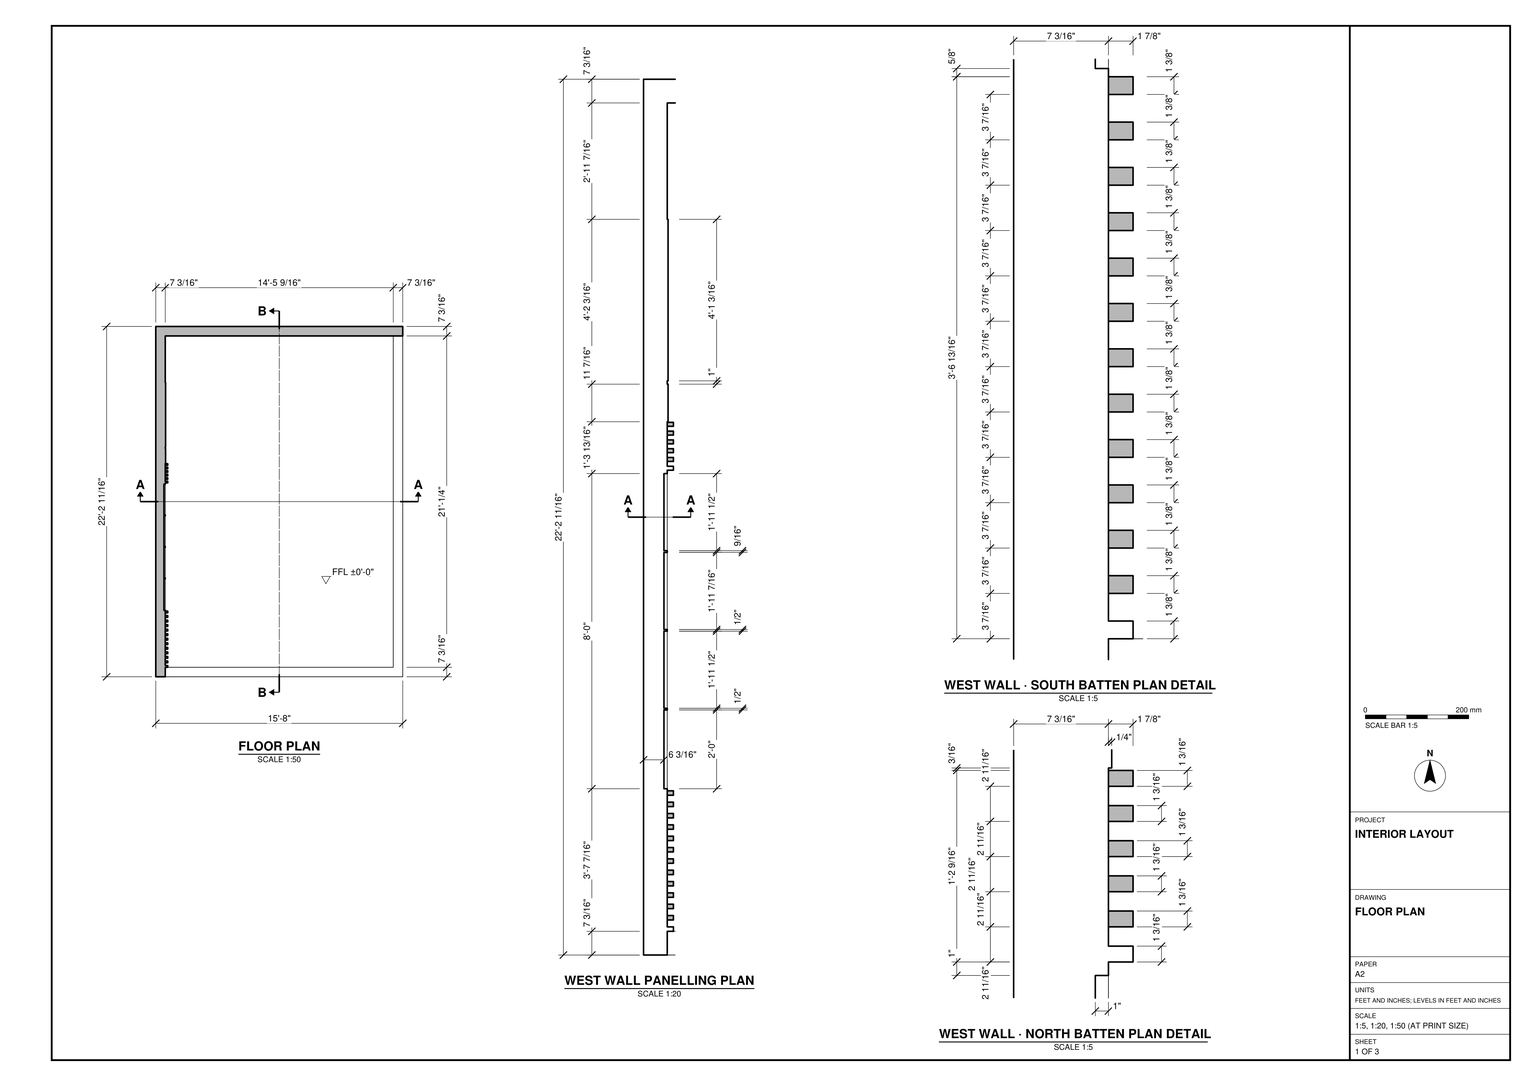
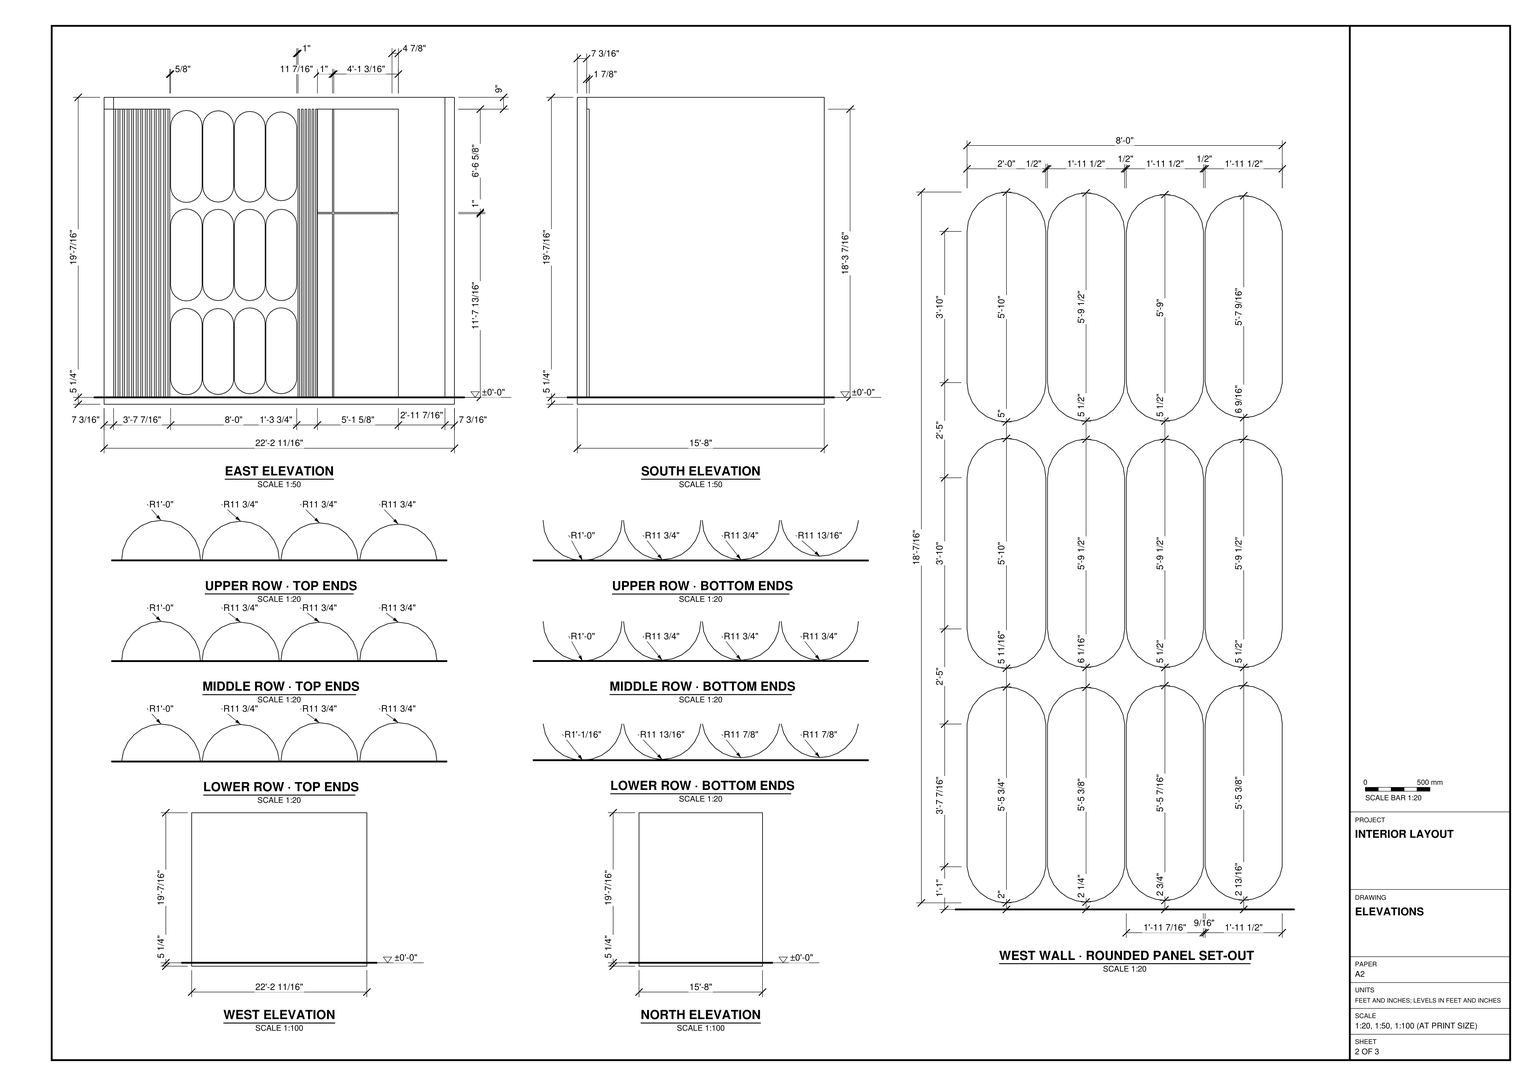
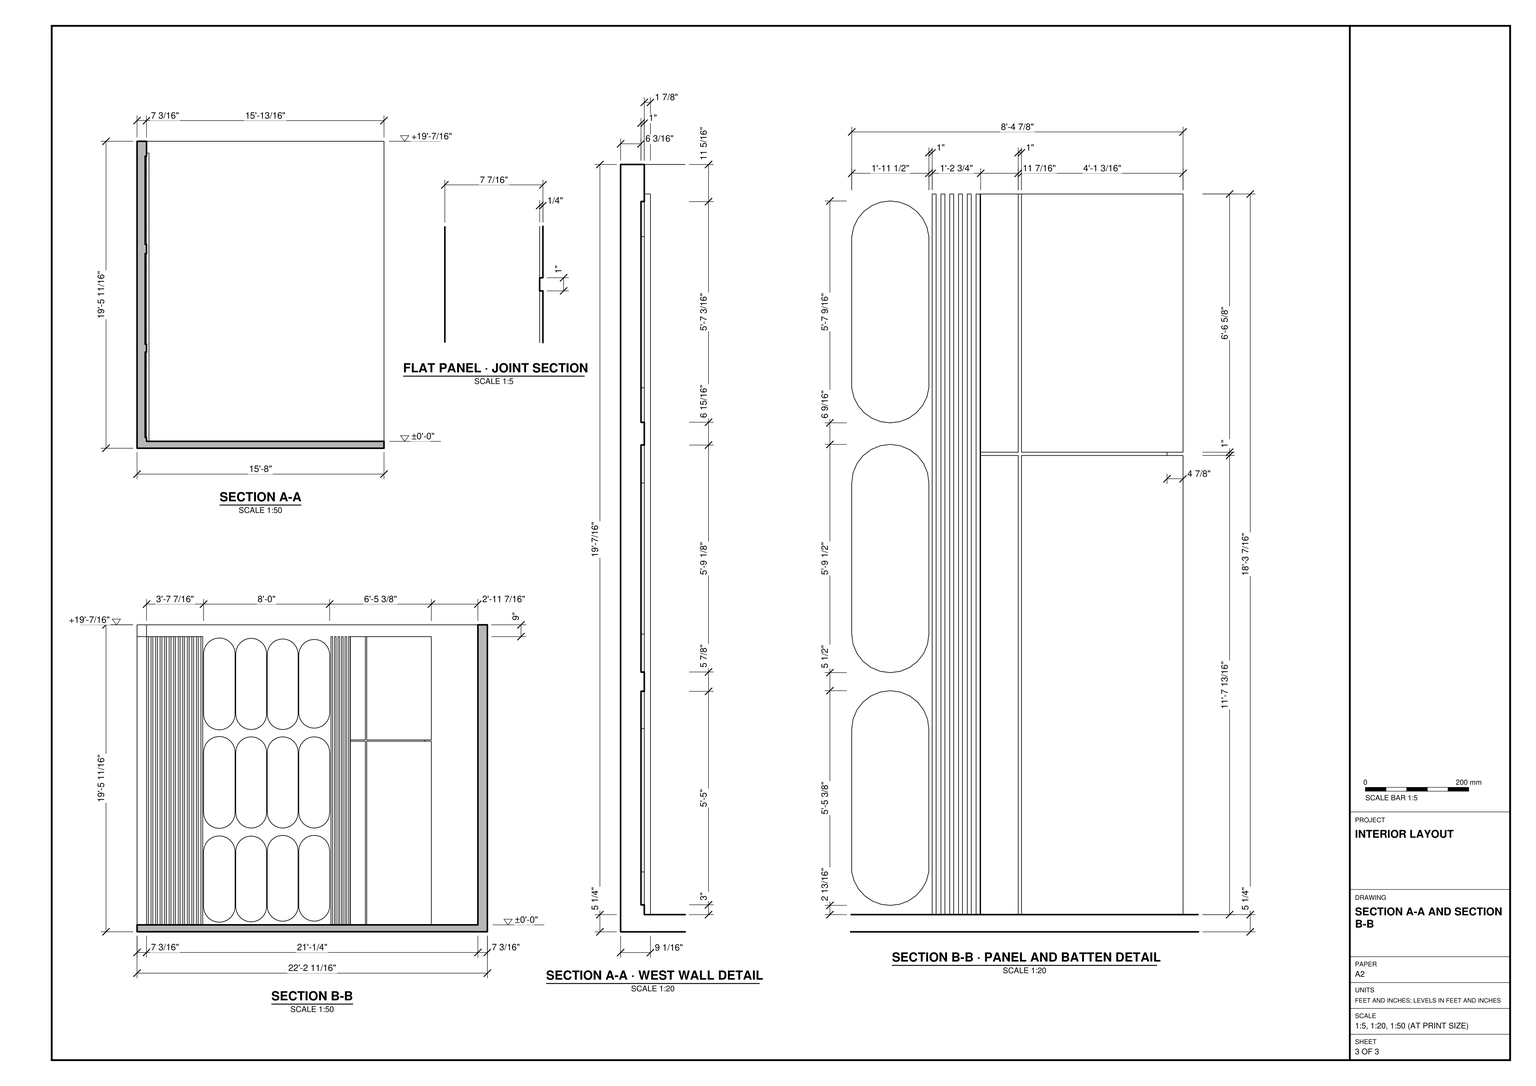
Build the interior shown in task_files/diagram_01.pdf in SketchUp. Work in feet and inches. Set the finished floor at ±0'-0" and model the rectangular slab with the west wall along its long edge and the north wall returning across its short edge. The overall dimensions are 15'-8" east to west, 22'-2 11/16" north to south and 19'-5 11/16" from the underside of the slab to the top of the walls. Make the slab 5 1/4" thick and use the 7 3/16" wall thickness shown in plan.

Set out the panelling on the room side of the west wall. Working from south to north, model the wider batten field, the rounded panels, the narrower batten field and the flat panels, leaving the plain wall face visible at the north end. Follow the separate plan details for the two batten spacings. Use the elevation to lay out the rounded ends in four columns and three rows, and use the sections to form the changes in face depth and the joints between flat panels.

Keep the slab, walls and built-in panelling in separate groups or components, and use components for repeated parts. Any decor or loose items shown may be suitable library components. Save one SketchUp model as output_files/interior_corner_with_detailed_west_wall_panelling.skp.

# SketchUp Ruby script. Lengths in inches.
U = 1.inch
M = Sketchup.active_model
def pt(a) = Geom::Point3d.new(a.map { |v| v * U })
def face(e, loops, mat)
  f = e.add_face(loops[0].map { |a| pt(a) })
  loops[1..].each { |l| e.add_face(l.map { |a| pt(a) }).erase! }
  f.material = f.back_material = mat if mat
  f
end
# faces: each face lists its corners as indices into pts; further lists are holes
def faces(e, pts, list, mat = nil) = list.each { |f| face(e, (f[0].is_a?(Array) ? f : [f]).map { |l| l.map { |i| pts[i] } }, mat) }
# xy, xz, yz: faces in a plane at the given z, y or x. An outline is a flat list of corners, or four numbers for a rectangle; further outlines are holes
def ring(l) = l.size == 4 ? [[l[0], l[1]], [l[2], l[1]], [l[2], l[3]], [l[0], l[3]]] : l.each_slice(2).to_a
def flat(e, list, mat, &to3) = list.each { |f| face(e, (f[0].is_a?(Array) ? f : [f]).map { |l| ring(l).map { |u, v| to3.(u, v) } }, mat) }
def xy(e, z, list, mat = nil) = flat(e, list, mat) { |x, y| [x, y, z] }
def xz(e, y, list, mat = nil) = flat(e, list, mat) { |x, z| [x, y, z] }
def yz(e, x, list, mat = nil) = flat(e, list, mat) { |y, z| [x, y, z] }
def lines(e, pts, list) = list.each { |a, b| e.add_line(pt(pts[a]), pt(pts[b])) }
# prism: a flat outline (further loops are holes) pulled along v
def prism(e, loops, v, mat = nil)
  f = face(e, loops, mat); d = Geom::Vector3d.new(v.map { |x| x * U })
  f.pushpull(f.normal.samedirection?(d) ? d.length : -d.length)
end
def box(e, o, s, mat = nil) = prism(e, [[o, [o[0] + s[0], o[1], o[2]], [o[0] + s[0], o[1] + s[1], o[2]], [o[0], o[1] + s[1], o[2]]]], [0, 0, s[2]], mat)
def at(x, y, z, deg = 0) = Geom::Transformation.translation(pt([x, y, z])) * Geom::Transformation.rotation(ORIGIN, Z_AXIS, deg.degrees)
def axes(o, x, y, z) = Geom::Transformation.new([*x, 0, *y, 0, *z, 0, *pt(o).to_a, 1])
def part(name) = M.definitions.add(name)
# library, detail: a bought-in or finely detailed component or shape, given as its bounding box
def library(name, o, s) = part(name).tap { |d| box(d.entities, o, s) }
def detail(e, o, s) = box(e.add_group.entities, o, s)
def put(e, d, t, mat = nil) = e.add_instance(d, t).tap { |i| i.material = mat if mat }
def group(e, t, mat = nil) = e.add_group.tap { |g| g.transformation = t; g.material = mat if mat }.entities
root = M.entities
xy(root,-2.9375,[[0,0,188,266.6875]])
xy(root,2.3125,[[7.22,0,188,0,188,259.47,180.78,259.47,180.78,7.22,7.22,7.22],[9.09,7.22,180.78,7.22,180.78,259.47,7.22,259.47,7.22,224.03,7.47,224.03,7.47,174.84,7.22,174.84,7.22,173.84,7.47,173.84,7.47,162.4,7.22,162.4,7.22,162.21,9.09,162.21,9.09,161,7.22,161,7.22,159.54,9.09,159.54,9.09,158.33,7.22,158.33,7.22,156.86,9.09,156.86,9.09,155.65,7.22,155.65,7.22,154.19,9.09,154.19,9.09,152.98,7.22,152.98,7.22,151.51,9.09,151.51,9.09,150.3,7.22,150.3,7.22,148.84,9.09,148.84,9.09,147.63,7.22,147.63,7.22,50,9.09,50,9.09,48.65,7.22,48.65,7.22,46.55,9.09,46.55,9.09,45.2,7.22,45.2,7.22,43.1,9.09,43.1,9.09,41.75,7.22,41.75,7.22,39.64,9.09,39.64,9.09,38.29,7.22,38.29,7.22,36.19,9.09,36.19,9.09,34.84,7.22,34.84,7.22,32.74,9.09,32.74,9.09,31.39,7.22,31.39,7.22,29.29,9.09,29.29,9.09,27.93,7.22,27.93,7.22,25.83,9.09,25.83,9.09,24.48,7.22,24.48,7.22,22.38,9.09,22.38,9.09,21.03,7.22,21.03,7.22,18.93,9.09,18.93,9.09,17.58,7.22,17.58,7.22,15.47,9.09,15.47,9.09,14.12,7.22,14.12,7.22,12.02,9.09,12.02,9.09,10.67,7.22,10.67,7.22,8.57,9.09,8.57],[7.22,10.67,9.09,12.02],[7.22,14.12,9.09,15.47],[7.22,17.58,9.09,18.93],
  [7.22,21.03,9.09,22.38],[7.22,24.48,9.09,25.83],[7.22,27.93,9.09,29.29],[7.22,31.39,9.09,32.74],[7.22,34.84,9.09,36.19],
  [7.22,38.29,9.09,39.64],[7.22,41.75,9.09,43.1],[7.22,45.2,9.09,46.55],[7.22,48.65,9.09,50]])
xy(root,142.125,[[7.22,162.4,7.47,173.84],[7.22,174.84,7.47,224.03]])
xy(root,143.125,[[7.22,162.4,7.47,173.84],[7.22,174.84,7.47,224.03]])
xy(root,221.75,[[7.22,7.22,9.09,8.57],[7.22,10.67,9.09,12.02],[7.22,14.12,9.09,15.47],[7.22,17.58,9.09,18.93],[7.22,21.03,9.09,22.38],
  [7.22,24.48,9.09,25.83],[7.22,27.93,9.09,29.29],[7.22,31.39,9.09,32.74],[7.22,34.84,9.09,36.19],[7.22,38.29,9.09,39.64],
  [7.22,41.75,9.09,43.1],[7.22,45.2,9.09,46.55],[7.22,48.65,9.09,50],[7.22,147.63,9.09,148.84],[7.22,150.3,9.09,151.51],
  [7.22,152.98,9.09,154.19],[7.22,155.65,9.09,156.86],[7.22,158.33,9.09,159.54],[7.22,161,9.09,162.21],[7.22,162.4,7.47,173.84],
  [7.22,174.84,7.47,224.03]])
xy(root,230.75,[[0,0,7.22,0,7.22,259.47,188,259.47,188,266.6875,0,266.6875]])
xz(root,0,[[0,-2.9375,188,-2.9375,188,2.3125,7.22,2.3125,7.22,230.75,0,230.75]])
xz(root,7.22,[[7.22,2.3125,9.09,221.75]])
xz(root,8.57,[[7.22,2.3125,9.09,221.75]])
xz(root,10.67,[[7.22,2.3125,9.09,221.75]])
xz(root,12.02,[[7.22,2.3125,9.09,221.75]])
xz(root,14.12,[[7.22,2.3125,9.09,221.75]])
xz(root,15.47,[[7.22,2.3125,9.09,221.75]])
xz(root,17.58,[[7.22,2.3125,9.09,221.75]])
xz(root,18.93,[[7.22,2.3125,9.09,221.75]])
xz(root,21.03,[[7.22,2.3125,9.09,221.75]])
xz(root,22.38,[[7.22,2.3125,9.09,221.75]])
xz(root,24.48,[[7.22,2.3125,9.09,221.75]])
xz(root,25.83,[[7.22,2.3125,9.09,221.75]])
xz(root,27.93,[[7.22,2.3125,9.09,221.75]])
xz(root,29.29,[[7.22,2.3125,9.09,221.75]])
xz(root,31.39,[[7.22,2.3125,9.09,221.75]])
xz(root,32.74,[[7.22,2.3125,9.09,221.75]])
xz(root,34.84,[[7.22,2.3125,9.09,221.75]])
xz(root,36.19,[[7.22,2.3125,9.09,221.75]])
xz(root,38.29,[[7.22,2.3125,9.09,221.75]])
xz(root,39.64,[[7.22,2.3125,9.09,221.75]])
xz(root,41.75,[[7.22,2.3125,9.09,221.75]])
xz(root,43.1,[[7.22,2.3125,9.09,221.75]])
xz(root,45.2,[[7.22,2.3125,9.09,221.75]])
xz(root,46.55,[[7.22,2.3125,9.09,221.75]])
xz(root,48.65,[[7.22,2.3125,9.09,221.75]])
xz(root,50,[[7.22,2.3125,9.09,221.75]])
xz(root,50.63,[[6.22,15.3125,7.22,58.75],[6.22,87.75,7.22,133.75],[6.22,162.75,7.22,208.76]])
xz(root,74.63,[[6.22,15.3125,7.22,58.75],[6.22,87.75,7.22,133.75],[6.22,162.75,7.22,208.76]])
xz(root,75.13,[[6.22,15.3125,7.22,58.75],[6.22,87.75,7.22,133.75],[6.22,162.75,7.22,208.76]])
xz(root,98.62,[[6.22,15.26,7.22,58.79],[6.22,58.79,7.22,58.82]])
xz(root,98.63,[[6.22,87.75,7.22,133.75],[6.22,162.75,7.22,208.76]])
xz(root,99.13,[[6.22,15.3125,7.22,58.75],[6.22,87.75,7.22,133.75],[6.22,162.75,7.22,208.76]])
xz(root,122.59,[[6.22,15.16,7.22,58.75]])
xz(root,122.63,[[6.22,87.75,7.22,133.75],[6.22,162.75,7.22,208.76]])
xz(root,123.13,[[6.22,15.3125,7.22,58.75],[6.22,87.75,7.22,133.75],[6.22,162.75,7.22,208.76]])
xz(root,146.6,[[6.22,15.3125,7.22,58.95]])
xz(root,146.63,[[6.22,87.75,7.22,133.75],[6.22,162.75,7.22,208.76]])
xz(root,147.63,[[7.22,2.3125,9.09,221.75]])
xz(root,148.84,[[7.22,2.3125,9.09,221.75]])
xz(root,150.3,[[7.22,2.3125,9.09,221.75]])
xz(root,151.51,[[7.22,2.3125,9.09,221.75]])
xz(root,152.98,[[7.22,2.3125,9.09,221.75]])
xz(root,154.19,[[7.22,2.3125,9.09,221.75]])
xz(root,155.65,[[7.22,2.3125,9.09,221.75]])
xz(root,156.86,[[7.22,2.3125,9.09,221.75]])
xz(root,158.33,[[7.22,2.3125,9.09,221.75]])
xz(root,159.54,[[7.22,2.3125,9.09,221.75]])
xz(root,161,[[7.22,2.3125,9.09,221.75]])
xz(root,162.21,[[7.22,2.3125,9.09,221.75]])
xz(root,162.4,[[7.22,2.3125,7.47,142.125],[7.22,143.125,7.47,221.75]])
xz(root,173.84,[[7.22,2.3125,7.47,142.125],[7.22,143.125,7.47,221.75]])
xz(root,174.84,[[7.22,2.3125,7.47,142.125],[7.22,143.125,7.47,221.75]])
xz(root,224.03,[[7.22,2.3125,7.47,142.125],[7.22,143.125,7.47,221.75]])
xz(root,259.47,[[7.22,2.3125,188,230.75]])
xz(root,266.6875,[[0,-2.9375,188,230.75]])
yz(root,0,[[0,-2.9375,266.6875,230.75]])
yz(root,6.22,[[62.63,4.3125,65.58,4.68,68.35,5.76,70.77,7.48,72.69,9.74,74.01,12.41,74.63,15.3125,74.63,58.75,74.07,61.72,72.79,64.46,70.875,66.79,68.43,68.57,65.625,69.68,62.63,70.0625,59.63,69.68,56.82,68.57,54.38,66.79,52.46,64.46,51.18,61.72,50.63,58.75,50.63,15.3125,51.25,12.41,52.5625,9.74,54.49,7.48,56.91,5.76,59.68,4.68],[86.88,4.5625,89.76,4.92,92.47,5.97,94.84,7.66,96.73,9.87,98.02,12.47,98.62,15.26,98.62,58.82,98.11,61.68,96.87,64.39,94.99,66.69,92.59,68.46,89.83,69.5625,86.88,69.9375,83.93,69.5625,81.16,68.46,78.77,66.69,76.89,64.39,75.65,61.68,75.13,58.75,75.13,15.3125,75.74,12.47,77.03,9.87,78.92,7.66,81.29,5.97,83.99,4.92],[110.88,5.0625,113.6875,5.4,116.34,6.39,118.68,7.99,120.57,10.09,121.91,12.58,122.59,15.16,122.59,58.75,122.19,61.79,121.02,64.62,119.15,67.04,116.72,68.91,113.9,70.08,110.86,70.48,107.82,70.08,104.99,68.91,102.56,67.04,100.7,64.62,99.53,61.79,99.13,58.75,99.13,15.3125,99.84,12.58,101.1875,10.09,103.08,7.99,105.42,6.39,108.07,5.4],[134.87,5.125,137.66,5.46,140.3,6.45,142.64,8.03,144.53,10.11,145.88,12.59,146.6,15.3125,146.6,58.95,146.23,61.79,145.05,64.625,143.1875,67.06,140.75,68.93,137.92,70.1,134.88,70.5,131.84,70.1,129,68.93,126.57,67.06,124.7,64.625,123.53,61.79,123.13,58.75,123.13,15.3125,123.85,12.59,125.2,10.11,127.09,8.03,129.43,6.45,132.07,5.46],[62.63,75.75,65.73,76.16,68.63,77.36,71.11,79.26,73.02,81.75,74.22,84.64,74.63,87.75,74.63,133.75,74.22,136.86,73.02,139.75,71.11,142.24,68.63,144.14,65.73,145.34,62.63,145.75,59.52,145.34,56.63,144.14,54.14,142.24,52.24,139.75,51.04,136.86,50.63,133.75,50.63,87.75,51.04,84.64,52.24,81.75,54.14,79.26,56.63,77.36,59.52,76.16],
  [86.88,76,89.92,76.4,92.75,77.57,95.1875,79.44,97.05,81.875,98.23,84.71,98.63,87.75,98.63,133.75,98.23,136.79,97.05,139.625,95.1875,142.06,92.75,143.93,89.92,145.1,86.88,145.5,83.84,145.1,81,143.93,78.57,142.06,76.7,139.625,75.53,136.79,75.13,133.75,75.13,87.75,75.53,84.71,76.7,81.875,78.57,79.44,81,77.57,83.84,76.4],[110.88,76,113.92,76.4,116.75,77.57,119.1875,79.44,121.05,81.875,122.23,84.71,122.63,87.75,122.63,133.75,122.23,136.79,121.05,139.625,119.1875,142.06,116.75,143.93,113.92,145.1,110.88,145.5,107.84,145.1,105,143.93,102.57,142.06,100.7,139.625,99.53,136.79,99.13,133.75,99.13,87.75,99.53,84.71,100.7,81.875,102.57,79.44,105,77.57,107.84,76.4],[134.88,76,137.92,76.4,140.75,77.57,143.1875,79.44,145.05,81.875,146.23,84.71,146.63,87.75,146.63,133.75,146.23,136.79,145.05,139.625,143.1875,142.06,140.75,143.93,137.92,145.1,134.88,145.5,131.84,145.1,129,143.93,126.57,142.06,124.7,139.625,123.53,136.79,123.13,133.75,123.13,87.75,123.53,84.71,124.7,81.875,126.57,79.44,129,77.57,131.84,76.4],[62.63,150.75,65.73,151.16,68.63,152.36,71.11,154.26,73.02,156.75,74.22,159.64,74.63,162.75,74.63,208.76,74.22,211.87,73.02,214.76,71.11,217.25,68.63,219.15,65.73,220.35,62.63,220.76,59.52,220.35,56.63,219.15,54.14,217.25,52.24,214.76,51.04,211.87,50.63,208.76,50.63,162.75,51.04,159.64,52.24,156.75,54.14,154.26,56.63,152.36,59.52,151.16],[86.88,151,89.92,151.4,92.75,152.57,95.1875,154.44,97.05,156.875,98.23,159.71,98.63,162.75,98.63,208.76,98.23,211.8,97.05,214.64,95.1875,217.07,92.75,218.9375,89.92,220.11,86.88,220.51,83.84,220.11,81,218.9375,78.57,217.07,76.7,214.64,75.53,211.8,75.13,208.76,75.13,162.75,75.53,159.71,76.7,156.875,78.57,154.44,81,152.57,83.84,151.4],
  [110.88,151,113.92,151.4,116.75,152.57,119.1875,154.44,121.05,156.875,122.23,159.71,122.63,162.75,122.63,208.76,122.12,211.7,120.89,214.42,119.01,216.74,116.61,218.52,113.84,219.63,110.88,220.01,107.92,219.63,105.15,218.52,102.75,216.74,100.87,214.42,99.64,211.7,99.13,208.76,99.13,162.75,99.53,159.71,100.7,156.875,102.57,154.44,105,152.57,107.84,151.4],[134.88,152.0625,137.75,152.42,140.45,153.46,142.82,155.13,144.71,157.33,146,159.92,146.63,162.75,146.63,208.76,146.04,211.625,144.77,214.26,142.88,216.5,140.51,218.2,137.78,219.27,134.88,219.64,131.98,219.27,129.25,218.2,126.875,216.5,124.99,214.26,123.72,211.625,123.13,208.76,123.13,162.75,123.75,159.92,125.05,157.33,126.9375,155.13,129.3,153.46,132,152.42]])
yz(root,7.22,[[0,2.3125,7.22,221.75],[[50,2.3125,147.63,2.3125,147.63,221.75,148.84,221.75,148.84,2.3125,150.3,2.3125,150.3,221.75,151.51,221.75,151.51,2.3125,152.98,2.3125,152.98,221.75,154.19,221.75,154.19,2.3125,155.65,2.3125,155.65,221.75,156.86,221.75,156.86,2.3125,158.33,2.3125,158.33,221.75,159.54,221.75,159.54,2.3125,161,2.3125,161,221.75,162.21,221.75,162.21,2.3125,162.4,2.3125,162.4,221.75,224.03,221.75,224.03,143.125,219.15,143.125,219.15,142.125,224.03,142.125,224.03,2.3125,259.47,2.3125,259.47,230.75,7.22,230.75,7.22,221.75,50,221.75],[62.63,150.75,59.52,151.16,56.63,152.36,54.14,154.26,52.24,156.75,51.04,159.64,50.63,162.75,50.63,208.76,51.04,211.87,52.24,214.76,54.14,217.25,56.63,219.15,59.52,220.35,62.63,220.76,65.73,220.35,68.63,219.15,71.11,217.25,73.02,214.76,74.22,211.87,74.63,208.76,74.63,162.75,74.22,159.64,73.02,156.75,71.11,154.26,68.63,152.36,65.73,151.16],[62.63,75.75,59.52,76.16,56.63,77.36,54.14,79.26,52.24,81.75,51.04,84.64,50.63,87.75,50.63,133.75,51.04,136.86,52.24,139.75,54.14,142.24,56.63,144.14,59.52,145.34,62.63,145.75,65.73,145.34,68.63,144.14,71.11,142.24,73.02,139.75,74.22,136.86,74.63,133.75,74.63,87.75,74.22,84.64,73.02,81.75,71.11,79.26,68.63,77.36,65.73,76.16],[86.88,151,83.84,151.4,81,152.57,78.57,154.44,76.7,156.875,75.53,159.71,75.13,162.75,75.13,208.76,75.53,211.8,76.7,214.64,78.57,217.07,81,218.9375,83.84,220.11,86.88,220.51,89.92,220.11,92.75,218.9375,95.1875,217.07,97.05,214.64,98.23,211.8,98.63,208.76,98.63,162.75,98.23,159.71,97.05,156.875,95.1875,154.44,92.75,152.57,89.92,151.4],[86.88,76,83.84,76.4,81,77.57,78.57,79.44,76.7,81.875,75.53,84.71,75.13,87.75,75.13,133.75,75.53,136.79,76.7,139.625,78.57,142.06,81,143.93,83.84,145.1,86.88,145.5,89.92,145.1,92.75,143.93,95.1875,142.06,97.05,139.625,98.23,136.79,98.63,133.75,98.63,87.75,98.23,84.71,97.05,81.875,95.1875,79.44,92.75,77.57,89.92,76.4],[110.88,76,107.84,76.4,105,77.57,102.57,79.44,100.7,81.875,99.53,84.71,99.13,87.75,99.13,133.75,99.53,136.79,100.7,139.625,102.57,142.06,105,143.93,107.84,145.1,110.88,145.5,113.92,145.1,116.75,143.93,119.1875,142.06,121.05,139.625,122.23,136.79,122.63,133.75,122.63,87.75,122.23,84.71,121.05,81.875,119.1875,79.44,116.75,77.57,113.92,76.4],[134.88,76,131.84,76.4,129,77.57,126.57,79.44,124.7,81.875,123.53,84.71,123.13,87.75,123.13,133.75,123.53,136.79,124.7,139.625,126.57,142.06,129,143.93,131.84,145.1,134.88,145.5,137.92,145.1,140.75,143.93,143.1875,142.06,145.05,139.625,146.23,136.79,146.63,133.75,146.63,87.75,146.23,84.71,145.05,81.875,143.1875,79.44,140.75,77.57,137.92,76.4],[110.88,151,107.84,151.4,105,152.57,102.57,154.44,100.7,156.875,99.53,159.71,99.13,162.75,99.13,208.76,99.64,211.7,100.87,214.42,102.75,216.74,105.15,218.52,107.92,219.63,110.88,220.01,113.84,219.63,116.61,218.52,119.01,216.74,120.89,214.42,122.12,211.7,122.63,208.76,122.63,162.75,122.23,159.71,121.05,156.875,119.1875,154.44,116.75,152.57,113.92,151.4],[134.88,152.0625,132,152.42,129.3,153.46,126.9375,155.13,125.05,157.33,123.75,159.92,123.13,162.75,123.13,208.76,123.72,211.625,124.99,214.26,126.875,216.5,129.25,218.2,131.98,219.27,134.88,219.64,137.78,219.27,140.51,218.2,142.88,216.5,144.77,214.26,146.04,211.625,146.63,208.76,146.63,162.75,146,159.92,144.71,157.33,142.82,155.13,140.45,153.46,137.75,152.42],[62.63,4.3125,59.68,4.68,56.91,5.76,54.49,7.48,52.5625,9.74,51.25,12.41,50.63,15.3125,50.63,58.75,51.18,61.72,52.46,64.46,54.38,66.79,56.82,68.57,59.63,69.68,62.63,70.0625,65.625,69.68,68.43,68.57,70.875,66.79,72.79,64.46,74.07,61.72,74.63,58.75,74.63,15.3125,74.01,12.41,72.69,9.74,70.77,7.48,68.35,5.76,65.58,4.68],[110.88,5.0625,108.07,5.4,105.42,6.39,103.08,7.99,101.1875,10.09,99.84,12.58,99.13,15.3125,99.13,58.75,99.53,61.79,100.7,64.62,102.56,67.04,104.99,68.91,107.82,70.08,110.86,70.48,113.9,70.08,116.72,68.91,119.15,67.04,121.02,64.62,122.19,61.79,122.59,58.75,122.59,15.16,121.91,12.58,120.57,10.09,118.68,7.99,116.34,6.39,113.6875,5.4],[86.88,4.5625,83.99,4.92,81.29,5.97,78.92,7.66,77.03,9.87,75.74,12.47,75.13,15.3125,75.13,58.75,75.65,61.68,76.89,64.39,78.77,66.69,81.16,68.46,83.93,69.5625,86.88,69.9375,89.83,69.5625,92.59,68.46,94.99,66.69,96.87,64.39,98.11,61.68,98.62,58.82,98.63,58.75,98.62,58.79,98.62,15.26,98.02,12.47,96.73,9.87,94.84,7.66,92.47,5.97,89.76,4.92],[134.87,5.125,132.07,5.46,129.43,6.45,127.09,8.03,125.2,10.11,123.85,12.59,123.13,15.3125,123.13,58.75,123.53,61.79,124.7,64.625,126.57,67.06,129,68.93,131.84,70.1,134.88,70.5,137.92,70.1,140.75,68.93,143.1875,67.06,145.05,64.625,146.23,61.79,146.6,58.95,146.6,15.3125,145.88,12.59,144.53,10.11,142.64,8.03,140.3,6.45,137.66,5.46]],[8.57,2.3125,10.67,221.75],[10.67,2.3125,12.02,221.75],[12.02,2.3125,14.12,221.75],
  [14.12,2.3125,15.47,221.75],[15.47,2.3125,17.58,221.75],[17.58,2.3125,18.93,221.75],[18.93,2.3125,21.03,221.75],[21.03,2.3125,22.38,221.75],
  [22.38,2.3125,24.48,221.75],[24.48,2.3125,25.83,221.75],[25.83,2.3125,27.93,221.75],[27.93,2.3125,29.29,221.75],[29.29,2.3125,31.39,221.75],
  [31.39,2.3125,32.74,221.75],[32.74,2.3125,34.84,221.75],[34.84,2.3125,36.19,221.75],[36.19,2.3125,38.29,221.75],[38.29,2.3125,39.64,221.75],
  [39.64,2.3125,41.75,221.75],[41.75,2.3125,43.1,221.75],[43.1,2.3125,45.2,221.75],[45.2,2.3125,46.55,221.75],[46.55,2.3125,48.65,221.75],
  [48.65,2.3125,50,221.75],[150.3,2.3125,151.51,221.75],[152.98,2.3125,154.19,221.75],[155.65,2.3125,156.86,221.75],[158.33,2.3125,159.54,221.75],
  [161,2.3125,162.21,221.75],[173.84,2.3125,174.84,2.3125,174.84,142.125,219.15,142.125,219.15,143.125,174.84,143.125,174.84,221.75,173.84,221.75,173.84,143.125,162.4,143.125,162.4,142.125,173.84,142.125],[98.63,58.75,98.62,58.82,98.62,58.79],[0,221.75,7.22,230.75]])
yz(root,7.47,[[162.4,2.3125,173.84,142.125],[174.84,2.3125,224.03,142.125],[162.4,143.125,173.84,221.75],[174.84,143.125,224.03,221.75]])
yz(root,9.09,[[7.22,2.3125,8.57,221.75],[10.67,2.3125,12.02,221.75],[14.12,2.3125,15.47,221.75],[17.58,2.3125,18.93,221.75],[21.03,2.3125,22.38,221.75],
  [24.48,2.3125,25.83,221.75],[27.93,2.3125,29.29,221.75],[31.39,2.3125,32.74,221.75],[34.84,2.3125,36.19,221.75],[38.29,2.3125,39.64,221.75],
  [41.75,2.3125,43.1,221.75],[45.2,2.3125,46.55,221.75],[48.65,2.3125,50,221.75],[147.63,2.3125,148.84,221.75],[150.3,2.3125,151.51,221.75],
  [152.98,2.3125,154.19,221.75],[155.65,2.3125,156.86,221.75],[158.33,2.3125,159.54,221.75],[161,2.3125,162.21,221.75]])
yz(root,188,[[0,-2.9375,266.6875,2.3125],[259.47,2.3125,266.6875,230.75]])
p = [[7.22,59.68,4.68],[7.22,62.63,4.3125],[6.22,62.63,4.3125],[6.22,59.68,4.68],[7.22,65.58,4.68],[6.22,65.58,4.68],
  [7.22,83.99,4.92],[7.22,86.88,4.5625],[6.22,86.88,4.5625],[6.22,83.99,4.92],[7.22,89.76,4.92],[6.22,89.76,4.92],
  [7.22,56.91,5.76],[6.22,56.91,5.76],[7.22,68.35,5.76],[6.22,68.35,5.76],[7.22,81.29,5.97],[6.22,81.29,5.97],
  [7.22,92.47,5.97],[6.22,92.47,5.97],[7.22,108.07,5.4],[7.22,110.88,5.0625],[6.22,110.88,5.0625],[6.22,108.07,5.4],
  [7.22,113.6875,5.4],[6.22,113.6875,5.4],[7.22,132.07,5.46],[7.22,134.87,5.125],[6.22,134.87,5.125],[6.22,132.07,5.46],
  [7.22,137.66,5.46],[6.22,137.66,5.46],[7.22,105.42,6.39],[6.22,105.42,6.39],[7.22,116.34,6.39],[6.22,116.34,6.39],
  [7.22,129.43,6.45],[6.22,129.43,6.45],[7.22,140.3,6.45],[6.22,140.3,6.45],[7.22,54.49,7.48],[6.22,54.49,7.48],
  [7.22,70.77,7.48],[6.22,70.77,7.48],[7.22,78.92,7.66],[6.22,78.92,7.66],[7.22,94.84,7.66],[6.22,94.84,7.66],
  [7.22,103.08,7.99],[6.22,103.08,7.99],[7.22,118.68,7.99],[6.22,118.68,7.99],[7.22,127.09,8.03],[6.22,127.09,8.03],
  [7.22,142.64,8.03],[6.22,142.64,8.03],[7.22,52.5625,9.74],[6.22,52.5625,9.74],[7.22,72.69,9.74],[6.22,72.69,9.74],
  [7.22,77.03,9.87],[6.22,77.03,9.87],[7.22,96.73,9.87],[6.22,96.73,9.87],[7.22,101.1875,10.09],[6.22,101.1875,10.09],
  [7.22,120.57,10.09],[6.22,120.57,10.09],[7.22,125.2,10.11],[6.22,125.2,10.11],[7.22,144.53,10.11],[6.22,144.53,10.11],
  [7.22,51.25,12.41],[6.22,51.25,12.41],[7.22,74.01,12.41],[6.22,74.01,12.41],[7.22,75.74,12.47],[6.22,75.74,12.47],
  [7.22,98.02,12.47],[6.22,98.02,12.47],[7.22,99.84,12.58],[6.22,99.84,12.58],[7.22,121.91,12.58],[6.22,121.91,12.58],
  [7.22,123.85,12.59],[6.22,123.85,12.59],[7.22,145.88,12.59],[6.22,145.88,12.59],[7.22,50.63,15.3125],[6.22,50.63,15.3125],
  [7.22,74.63,15.3125],[6.22,74.63,15.3125],[7.22,75.13,15.3125],[6.22,75.13,15.3125],[7.22,98.62,15.26],[6.22,98.62,15.26],
  [7.22,99.13,15.3125],[6.22,99.13,15.3125],[7.22,122.59,15.16],[6.22,122.59,15.16],[7.22,123.13,15.3125],[6.22,123.13,15.3125],
  [7.22,146.6,15.3125],[6.22,146.6,15.3125],[7.22,74.63,58.75],[7.22,74.07,61.72],[6.22,74.07,61.72],[6.22,74.63,58.75],
  [7.22,122.59,58.75],[7.22,122.19,61.79],[6.22,122.19,61.79],[6.22,122.59,58.75],[7.22,51.18,61.72],[7.22,50.63,58.75],
  [6.22,50.63,58.75],[6.22,51.18,61.72],[7.22,75.65,61.68],[7.22,75.13,58.75],[6.22,75.13,58.75],[6.22,75.65,61.68],
  [7.22,98.62,58.82],[7.22,98.11,61.68],[6.22,98.11,61.68],[6.22,98.62,58.82],[7.22,99.53,61.79],[7.22,99.13,58.75],
  [6.22,99.13,58.75],[6.22,99.53,61.79],[7.22,123.53,61.79],[7.22,123.13,58.75],[6.22,123.13,58.75],[6.22,123.53,61.79],
  [7.22,146.6,58.95],[7.22,146.23,61.79],[6.22,146.23,61.79],[6.22,146.6,58.95],[7.22,52.46,64.46],[6.22,52.46,64.46],
  [7.22,72.79,64.46],[6.22,72.79,64.46],[7.22,76.89,64.39],[6.22,76.89,64.39],[7.22,96.87,64.39],[6.22,96.87,64.39],
  [7.22,100.7,64.62],[6.22,100.7,64.62],[7.22,121.02,64.62],[6.22,121.02,64.62],[7.22,124.7,64.625],[6.22,124.7,64.625],
  [7.22,145.05,64.625],[6.22,145.05,64.625],[7.22,78.77,66.69],[6.22,78.77,66.69],[7.22,94.99,66.69],[6.22,94.99,66.69],
  [7.22,54.38,66.79],[6.22,54.38,66.79],[7.22,70.875,66.79],[6.22,70.875,66.79],[7.22,102.56,67.04],[6.22,102.56,67.04],
  [7.22,119.15,67.04],[6.22,119.15,67.04],[7.22,126.57,67.06],[6.22,126.57,67.06],[7.22,143.1875,67.06],[6.22,143.1875,67.06],
  [7.22,81.16,68.46],[6.22,81.16,68.46],[7.22,92.59,68.46],[6.22,92.59,68.46],[7.22,56.82,68.57],[6.22,56.82,68.57],
  [7.22,68.43,68.57],[6.22,68.43,68.57],[7.22,104.99,68.91],[6.22,104.99,68.91],[7.22,116.72,68.91],[6.22,116.72,68.91],
  [7.22,129,68.93],[6.22,129,68.93],[7.22,140.75,68.93],[6.22,140.75,68.93],[7.22,83.93,69.5625],[6.22,83.93,69.5625],
  [7.22,89.83,69.5625],[6.22,89.83,69.5625],[7.22,59.63,69.68],[6.22,59.63,69.68],[7.22,65.625,69.68],[6.22,65.625,69.68],
  [7.22,107.82,70.08],[6.22,107.82,70.08],[7.22,113.9,70.08],[6.22,113.9,70.08],[7.22,131.84,70.1],[6.22,131.84,70.1],
  [7.22,137.92,70.1],[6.22,137.92,70.1],[7.22,86.88,69.9375],[6.22,86.88,69.9375],[7.22,62.63,70.0625],[6.22,62.63,70.0625],
  [7.22,110.86,70.48],[6.22,110.86,70.48],[7.22,134.88,70.5],[6.22,134.88,70.5],[7.22,59.52,76.16],[7.22,62.63,75.75],
  [6.22,62.63,75.75],[6.22,59.52,76.16],[7.22,65.73,76.16],[6.22,65.73,76.16],[7.22,83.84,76.4],[7.22,86.88,76],
  [6.22,86.88,76],[6.22,83.84,76.4],[7.22,89.92,76.4],[6.22,89.92,76.4],[7.22,107.84,76.4],[7.22,110.88,76],
  [6.22,110.88,76],[6.22,107.84,76.4],[7.22,113.92,76.4],[6.22,113.92,76.4],[7.22,131.84,76.4],[7.22,134.88,76],
  [6.22,134.88,76],[6.22,131.84,76.4],[7.22,137.92,76.4],[6.22,137.92,76.4],[7.22,56.63,77.36],[6.22,56.63,77.36],
  [7.22,68.63,77.36],[6.22,68.63,77.36],[7.22,81,77.57],[6.22,81,77.57],[7.22,92.75,77.57],[6.22,92.75,77.57],
  [7.22,105,77.57],[6.22,105,77.57],[7.22,116.75,77.57],[6.22,116.75,77.57],[7.22,129,77.57],[6.22,129,77.57],
  [7.22,140.75,77.57],[6.22,140.75,77.57],[7.22,54.14,79.26],[6.22,54.14,79.26],[7.22,71.11,79.26],[6.22,71.11,79.26],
  [7.22,78.57,79.44],[6.22,78.57,79.44],[7.22,95.1875,79.44],[6.22,95.1875,79.44],[7.22,102.57,79.44],[6.22,102.57,79.44],
  [7.22,119.1875,79.44],[6.22,119.1875,79.44],[7.22,126.57,79.44],[6.22,126.57,79.44],[7.22,143.1875,79.44],[6.22,143.1875,79.44],
  [7.22,52.24,81.75],[6.22,52.24,81.75],[7.22,73.02,81.75],[6.22,73.02,81.75],[7.22,76.7,81.875],[6.22,76.7,81.875],
  [7.22,97.05,81.875],[6.22,97.05,81.875],[7.22,100.7,81.875],[6.22,100.7,81.875],[7.22,121.05,81.875],[6.22,121.05,81.875],
  [7.22,124.7,81.875],[6.22,124.7,81.875],[7.22,145.05,81.875],[6.22,145.05,81.875],[7.22,51.04,84.64],[6.22,51.04,84.64],
  [7.22,74.22,84.64],[6.22,74.22,84.64],[7.22,75.53,84.71],[6.22,75.53,84.71],[7.22,98.23,84.71],[6.22,98.23,84.71],
  [7.22,99.53,84.71],[6.22,99.53,84.71],[7.22,122.23,84.71],[6.22,122.23,84.71],[7.22,123.53,84.71],[6.22,123.53,84.71],
  [7.22,146.23,84.71],[6.22,146.23,84.71],[7.22,50.63,87.75],[6.22,50.63,87.75],[7.22,74.63,87.75],[6.22,74.63,87.75],
  [7.22,75.13,87.75],[6.22,75.13,87.75],[7.22,98.63,87.75],[6.22,98.63,87.75],[7.22,99.13,87.75],[6.22,99.13,87.75],
  [7.22,122.63,87.75],[6.22,122.63,87.75],[7.22,123.13,87.75],[6.22,123.13,87.75],[7.22,146.63,87.75],[6.22,146.63,87.75],
  [7.22,51.04,136.86],[7.22,50.63,133.75],[6.22,50.63,133.75],[6.22,51.04,136.86],[7.22,74.63,133.75],[7.22,74.22,136.86],
  [6.22,74.22,136.86],[6.22,74.63,133.75],[7.22,75.53,136.79],[7.22,75.13,133.75],[6.22,75.13,133.75],[6.22,75.53,136.79],
  [7.22,98.63,133.75],[7.22,98.23,136.79],[6.22,98.23,136.79],[6.22,98.63,133.75],[7.22,99.53,136.79],[7.22,99.13,133.75],
  [6.22,99.13,133.75],[6.22,99.53,136.79],[7.22,122.63,133.75],[7.22,122.23,136.79],[6.22,122.23,136.79],[6.22,122.63,133.75],
  [7.22,123.53,136.79],[7.22,123.13,133.75],[6.22,123.13,133.75],[6.22,123.53,136.79],[7.22,146.63,133.75],[7.22,146.23,136.79],
  [6.22,146.23,136.79],[6.22,146.63,133.75],[7.22,76.7,139.625],[6.22,76.7,139.625],[7.22,97.05,139.625],[6.22,97.05,139.625],
  [7.22,100.7,139.625],[6.22,100.7,139.625],[7.22,121.05,139.625],[6.22,121.05,139.625],[7.22,124.7,139.625],[6.22,124.7,139.625],
  [7.22,145.05,139.625],[6.22,145.05,139.625],[7.22,52.24,139.75],[6.22,52.24,139.75],[7.22,73.02,139.75],[6.22,73.02,139.75],
  [7.22,78.57,142.06],[6.22,78.57,142.06],[7.22,95.1875,142.06],[6.22,95.1875,142.06],[7.22,102.57,142.06],[6.22,102.57,142.06],
  [7.22,119.1875,142.06],[6.22,119.1875,142.06],[7.22,126.57,142.06],[6.22,126.57,142.06],[7.22,143.1875,142.06],[6.22,143.1875,142.06],
  [7.22,54.14,142.24],[6.22,54.14,142.24],[7.22,71.11,142.24],[6.22,71.11,142.24],[7.22,81,143.93],[6.22,81,143.93],
  [7.22,92.75,143.93],[6.22,92.75,143.93],[7.22,105,143.93],[6.22,105,143.93],[7.22,116.75,143.93],[6.22,116.75,143.93],
  [7.22,129,143.93],[6.22,129,143.93],[7.22,140.75,143.93],[6.22,140.75,143.93],[7.22,56.63,144.14],[6.22,56.63,144.14],
  [7.22,68.63,144.14],[6.22,68.63,144.14],[7.22,83.84,145.1],[6.22,83.84,145.1],[7.22,89.92,145.1],[6.22,89.92,145.1],
  [7.22,107.84,145.1],[6.22,107.84,145.1],[7.22,113.92,145.1],[6.22,113.92,145.1],[7.22,131.84,145.1],[6.22,131.84,145.1],
  [7.22,137.92,145.1],[6.22,137.92,145.1],[7.22,59.52,145.34],[6.22,59.52,145.34],[7.22,65.73,145.34],[6.22,65.73,145.34],
  [7.22,86.88,145.5],[6.22,86.88,145.5],[7.22,110.88,145.5],[6.22,110.88,145.5],[7.22,134.88,145.5],[6.22,134.88,145.5],
  [7.22,62.63,145.75],[6.22,62.63,145.75],[7.22,59.52,151.16],[7.22,62.63,150.75],[6.22,62.63,150.75],[6.22,59.52,151.16],
  [7.22,65.73,151.16],[6.22,65.73,151.16],[7.22,83.84,151.4],[7.22,86.88,151],[6.22,86.88,151],[6.22,83.84,151.4],
  [7.22,89.92,151.4],[6.22,89.92,151.4],[7.22,107.84,151.4],[7.22,110.88,151],[6.22,110.88,151],[6.22,107.84,151.4],
  [7.22,113.92,151.4],[6.22,113.92,151.4],[7.22,56.63,152.36],[6.22,56.63,152.36],[7.22,68.63,152.36],[6.22,68.63,152.36],
  [7.22,81,152.57],[6.22,81,152.57],[7.22,92.75,152.57],[6.22,92.75,152.57],[7.22,105,152.57],[6.22,105,152.57],
  [7.22,116.75,152.57],[6.22,116.75,152.57],[7.22,132,152.42],[7.22,134.88,152.0625],[6.22,134.88,152.0625],[6.22,132,152.42],
  [7.22,137.75,152.42],[6.22,137.75,152.42],[7.22,54.14,154.26],[6.22,54.14,154.26],[7.22,71.11,154.26],[6.22,71.11,154.26],
  [7.22,129.3,153.46],[6.22,129.3,153.46],[7.22,140.45,153.46],[6.22,140.45,153.46],[7.22,78.57,154.44],[6.22,78.57,154.44],
  [7.22,95.1875,154.44],[6.22,95.1875,154.44],[7.22,102.57,154.44],[6.22,102.57,154.44],[7.22,119.1875,154.44],[6.22,119.1875,154.44],
  [7.22,126.9375,155.13],[6.22,126.9375,155.13],[7.22,142.82,155.13],[6.22,142.82,155.13],[7.22,52.24,156.75],[6.22,52.24,156.75],
  [7.22,73.02,156.75],[6.22,73.02,156.75],[7.22,76.7,156.875],[6.22,76.7,156.875],[7.22,97.05,156.875],[6.22,97.05,156.875],
  [7.22,100.7,156.875],[6.22,100.7,156.875],[7.22,121.05,156.875],[6.22,121.05,156.875],[7.22,125.05,157.33],[6.22,125.05,157.33],
  [7.22,144.71,157.33],[6.22,144.71,157.33],[7.22,51.04,159.64],[6.22,51.04,159.64],[7.22,74.22,159.64],[6.22,74.22,159.64],
  [7.22,75.53,159.71],[6.22,75.53,159.71],[7.22,98.23,159.71],[6.22,98.23,159.71],[7.22,99.53,159.71],[6.22,99.53,159.71],
  [7.22,122.23,159.71],[6.22,122.23,159.71],[7.22,123.75,159.92],[6.22,123.75,159.92],[7.22,146,159.92],[6.22,146,159.92],
  [7.22,50.63,162.75],[6.22,50.63,162.75],[7.22,74.63,162.75],[6.22,74.63,162.75],[7.22,75.13,162.75],[6.22,75.13,162.75],
  [7.22,98.63,162.75],[6.22,98.63,162.75],[7.22,99.13,162.75],[6.22,99.13,162.75],[7.22,122.63,162.75],[6.22,122.63,162.75],
  [7.22,123.13,162.75],[6.22,123.13,162.75],[7.22,146.63,162.75],[6.22,146.63,162.75],[7.22,51.04,211.87],[7.22,50.63,208.76],
  [6.22,50.63,208.76],[6.22,51.04,211.87],[7.22,74.63,208.76],[7.22,74.22,211.87],[6.22,74.22,211.87],[6.22,74.63,208.76],
  [7.22,75.53,211.8],[7.22,75.13,208.76],[6.22,75.13,208.76],[6.22,75.53,211.8],[7.22,98.63,208.76],[7.22,98.23,211.8],
  [6.22,98.23,211.8],[6.22,98.63,208.76],[7.22,99.64,211.7],[7.22,99.13,208.76],[6.22,99.13,208.76],[6.22,99.64,211.7],
  [7.22,122.63,208.76],[7.22,122.12,211.7],[6.22,122.12,211.7],[6.22,122.63,208.76],[7.22,123.72,211.625],[7.22,123.13,208.76],
  [6.22,123.13,208.76],[6.22,123.72,211.625],[7.22,146.63,208.76],[7.22,146.04,211.625],[6.22,146.04,211.625],[6.22,146.63,208.76],
  [7.22,124.99,214.26],[6.22,124.99,214.26],[7.22,144.77,214.26],[6.22,144.77,214.26],[7.22,100.87,214.42],[6.22,100.87,214.42],
  [7.22,120.89,214.42],[6.22,120.89,214.42],[7.22,76.7,214.64],[6.22,76.7,214.64],[7.22,97.05,214.64],[6.22,97.05,214.64],
  [7.22,52.24,214.76],[6.22,52.24,214.76],[7.22,73.02,214.76],[6.22,73.02,214.76],[7.22,126.875,216.5],[6.22,126.875,216.5],
  [7.22,142.88,216.5],[6.22,142.88,216.5],[7.22,102.75,216.74],[6.22,102.75,216.74],[7.22,119.01,216.74],[6.22,119.01,216.74],
  [7.22,78.57,217.07],[6.22,78.57,217.07],[7.22,95.1875,217.07],[6.22,95.1875,217.07],[7.22,54.14,217.25],[6.22,54.14,217.25],
  [7.22,71.11,217.25],[6.22,71.11,217.25],[7.22,129.25,218.2],[6.22,129.25,218.2],[7.22,140.51,218.2],[6.22,140.51,218.2],
  [7.22,105.15,218.52],[6.22,105.15,218.52],[7.22,116.61,218.52],[6.22,116.61,218.52],[7.22,81,218.9375],[6.22,81,218.9375],
  [7.22,92.75,218.9375],[6.22,92.75,218.9375],[7.22,56.63,219.15],[6.22,56.63,219.15],[7.22,68.63,219.15],[6.22,68.63,219.15],
  [7.22,131.98,219.27],[6.22,131.98,219.27],[7.22,137.78,219.27],[6.22,137.78,219.27],[7.22,107.92,219.63],[6.22,107.92,219.63],
  [7.22,113.84,219.63],[6.22,113.84,219.63],[7.22,83.84,220.11],[6.22,83.84,220.11],[7.22,89.92,220.11],[6.22,89.92,220.11],
  [7.22,59.52,220.35],[6.22,59.52,220.35],[7.22,65.73,220.35],[6.22,65.73,220.35],[7.22,134.88,219.64],[6.22,134.88,219.64],
  [7.22,110.88,220.01],[6.22,110.88,220.01],[7.22,86.88,220.51],[6.22,86.88,220.51],[7.22,62.63,220.76],[6.22,62.63,220.76],
  [7.22,98.63,15.3125],[7.22,122.63,15.3125],[7.22,146.63,58.75]]
faces(root,p,[[0,1,2,3],[1,4,5,2],[6,7,8,9],[7,10,11,8],[12,0,3,13],[4,14,15,5],[16,6,9,17],[10,18,19,11],
  [20,21,22,23],[21,24,25,22],[26,27,28,29],[27,30,31,28],[32,20,23,33],[24,34,35,25],[36,26,29,37],[30,38,39,31],
  [40,12,13,41],[14,42,43,15],[44,16,17,45],[18,46,47,19],[48,32,33,49],[34,50,51,35],[52,36,37,53],[38,54,55,39],
  [56,40,41,57],[42,58,59,43],[60,44,45,61],[46,62,63,47],[64,48,49,65],[50,66,67,51],[68,52,53,69],[54,70,71,55],
  [72,56,57,73],[58,74,75,59],[76,60,61,77],[62,78,79,63],[80,64,65,81],[66,82,83,67],[84,68,69,85],[70,86,87,71],
  [88,72,73,89],[74,90,91,75],[92,76,77,93],[78,94,95,79],[96,80,81,97],[82,98,99,83],[100,84,85,101],[86,102,103,87],
  [104,105,106,107],[108,109,110,111],[112,113,114,115],[116,117,118,119],[120,121,122,123],[124,125,126,127],[128,129,130,131],[132,133,134,135],
  [136,112,115,137],[105,138,139,106],[140,116,119,141],[121,142,143,122],[144,124,127,145],[109,146,147,110],[148,128,131,149],[133,150,151,134],
  [152,140,141,153],[142,154,155,143],[156,136,137,157],[138,158,159,139],[160,144,145,161],[146,162,163,147],[164,148,149,165],[150,166,167,151],
  [168,152,153,169],[154,170,171,155],[172,156,157,173],[158,174,175,159],[176,160,161,177],[162,178,179,163],[180,164,165,181],[166,182,183,167],
  [184,168,169,185],[170,186,187,171],[188,172,173,189],[174,190,191,175],[192,176,177,193],[178,194,195,179],[196,180,181,197],[182,198,199,183],
  [200,184,185,201],[186,200,201,187],[202,188,189,203],[190,202,203,191],[204,192,193,205],[194,204,205,195],[206,196,197,207],[198,206,207,199],
  [208,209,210,211],[209,212,213,210],[214,215,216,217],[215,218,219,216],[220,221,222,223],[221,224,225,222],[226,227,228,229],[227,230,231,228],
  [232,208,211,233],[212,234,235,213],[236,214,217,237],[218,238,239,219],[240,220,223,241],[224,242,243,225],[244,226,229,245],[230,246,247,231],
  [248,232,233,249],[234,250,251,235],[252,236,237,253],[238,254,255,239],[256,240,241,257],[242,258,259,243],[260,244,245,261],[246,262,263,247],
  [264,248,249,265],[250,266,267,251],[268,252,253,269],[254,270,271,255],[272,256,257,273],[258,274,275,259],[276,260,261,277],[262,278,279,263],
  [280,264,265,281],[266,282,283,267],[284,268,269,285],[270,286,287,271],[288,272,273,289],[274,290,291,275],[292,276,277,293],[278,294,295,279],
  [296,280,281,297],[282,298,299,283],[300,284,285,301],[286,302,303,287],[304,288,289,305],[290,306,307,291],[308,292,293,309],[294,310,311,295],
  [312,313,314,315],[316,317,318,319],[320,321,322,323],[324,325,326,327],[328,329,330,331],[332,333,334,335],[336,337,338,339],[340,341,342,343],
  [344,320,323,345],[325,346,347,326],[348,328,331,349],[333,350,351,334],[352,336,339,353],[341,354,355,342],[356,312,315,357],[317,358,359,318],
  [360,344,345,361],[346,362,363,347],[364,348,349,365],[350,366,367,351],[368,352,353,369],[354,370,371,355],[372,356,357,373],[358,374,375,359],
  [376,360,361,377],[362,378,379,363],[380,364,365,381],[366,382,383,367],[384,368,369,385],[370,386,387,371],[388,372,373,389],[374,390,391,375],
  [392,376,377,393],[378,394,395,379],[396,380,381,397],[382,398,399,383],[400,384,385,401],[386,402,403,387],[404,388,389,405],[390,406,407,391],
  [408,392,393,409],[394,408,409,395],[410,396,397,411],[398,410,411,399],[412,400,401,413],[402,412,413,403],[414,404,405,415],[406,414,415,407],
  [416,417,418,419],[417,420,421,418],[422,423,424,425],[423,426,427,424],[428,429,430,431],[429,432,433,430],[434,416,419,435],[420,436,437,421],
  [438,422,425,439],[426,440,441,427],[442,428,431,443],[432,444,445,433],[446,447,448,449],[447,450,451,448],[452,434,435,453],[436,454,455,437],
  [456,446,449,457],[450,458,459,451],[460,438,439,461],[440,462,463,441],[464,442,443,465],[444,466,467,445],[468,456,457,469],[458,470,471,459],
  [472,452,453,473],[454,474,475,455],[476,460,461,477],[462,478,479,463],[480,464,465,481],[466,482,483,467],[484,468,469,485],[470,486,487,471],
  [488,472,473,489],[474,490,491,475],[492,476,477,493],[478,494,495,479],[496,480,481,497],[482,498,499,483],[500,484,485,501],[486,502,503,487],
  [504,488,489,505],[490,506,507,491],[508,492,493,509],[494,510,511,495],[512,496,497,513],[498,514,515,499],[516,500,501,517],[502,518,519,503],
  [520,521,522,523],[524,525,526,527],[528,529,530,531],[532,533,534,535],[536,537,538,539],[540,541,542,543],[544,545,546,547],[548,549,550,551],
  [552,544,547,553],[549,554,555,550],[556,536,539,557],[541,558,559,542],[560,528,531,561],[533,562,563,534],[564,520,523,565],[525,566,567,526],
  [568,552,553,569],[554,570,571,555],[572,556,557,573],[558,574,575,559],[576,560,561,577],[562,578,579,563],[580,564,565,581],[566,582,583,567],
  [584,568,569,585],[570,586,587,571],[588,572,573,589],[574,590,591,575],[592,576,577,593],[578,594,595,579],[596,580,581,597],[582,598,599,583],
  [600,584,585,601],[586,602,603,587],[604,588,589,605],[590,606,607,591],[608,592,593,609],[594,610,611,595],[612,596,597,613],[598,614,615,599],
  [616,600,601,617],[602,616,617,603],[618,604,605,619],[606,618,619,607],[620,608,609,621],[610,620,621,611],[622,612,613,623],[614,622,623,615]])
lines(root,p,[[94,624],[98,625],[132,626]])
